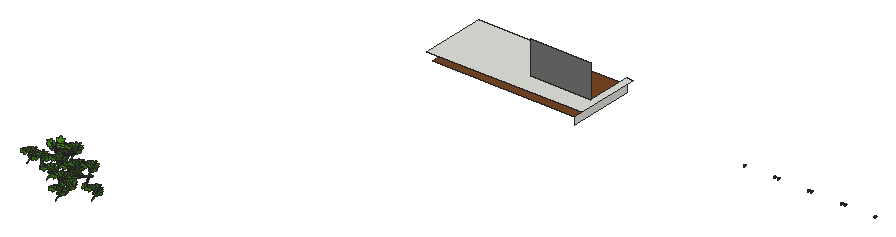
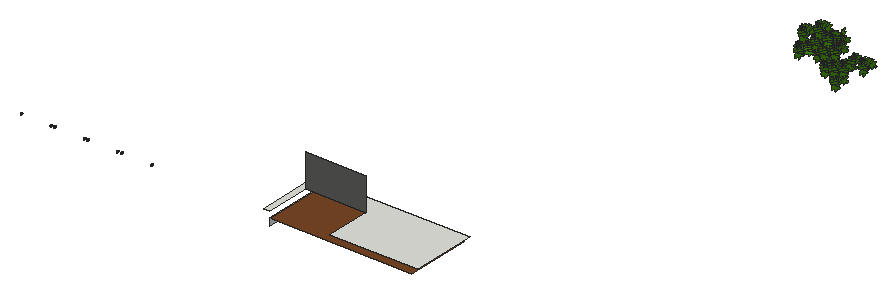
# SketchUp Ruby script. Lengths in inches.
U = 1.inch
M = Sketchup.active_model
def pt(a) = Geom::Point3d.new(a.map { |v| v * U })
def face(e, loops, mat)
  f = e.add_face(loops[0].map { |a| pt(a) })
  loops[1..].each { |l| e.add_face(l.map { |a| pt(a) }).erase! }
  f.material = f.back_material = mat if mat
  f
end
# faces: each face lists its corners as indices into pts; further lists are holes
def faces(e, pts, list, mat = nil) = list.each { |f| face(e, (f[0].is_a?(Array) ? f : [f]).map { |l| l.map { |i| pts[i] } }, mat) }
# xy, xz, yz: faces in a plane at the given z, y or x. An outline is a flat list of corners, or four numbers for a rectangle; further outlines are holes
def ring(l) = l.size == 4 ? [[l[0], l[1]], [l[2], l[1]], [l[2], l[3]], [l[0], l[3]]] : l.each_slice(2).to_a
def flat(e, list, mat, &to3) = list.each { |f| face(e, (f[0].is_a?(Array) ? f : [f]).map { |l| ring(l).map { |u, v| to3.(u, v) } }, mat) }
def xy(e, z, list, mat = nil) = flat(e, list, mat) { |x, y| [x, y, z] }
def xz(e, y, list, mat = nil) = flat(e, list, mat) { |x, z| [x, y, z] }
def yz(e, x, list, mat = nil) = flat(e, list, mat) { |y, z| [x, y, z] }
def lines(e, pts, list) = list.each { |a, b| e.add_line(pt(pts[a]), pt(pts[b])) }
# prism: a flat outline (further loops are holes) pulled along v
def prism(e, loops, v, mat = nil)
  f = face(e, loops, mat); d = Geom::Vector3d.new(v.map { |x| x * U })
  f.pushpull(f.normal.samedirection?(d) ? d.length : -d.length)
end
def box(e, o, s, mat = nil) = prism(e, [[o, [o[0] + s[0], o[1], o[2]], [o[0] + s[0], o[1] + s[1], o[2]], [o[0], o[1] + s[1], o[2]]]], [0, 0, s[2]], mat)
def at(x, y, z, deg = 0) = Geom::Transformation.translation(pt([x, y, z])) * Geom::Transformation.rotation(ORIGIN, Z_AXIS, deg.degrees)
def axes(o, x, y, z) = Geom::Transformation.new([*x, 0, *y, 0, *z, 0, *pt(o).to_a, 1])
def part(name) = M.definitions.add(name)
# library, detail: a bought-in or finely detailed component or shape, given as its bounding box
def library(name, o, s) = part(name).tap { |d| box(d.entities, o, s) }
def detail(e, o, s) = box(e.add_group.entities, o, s)
def put(e, d, t, mat = nil) = e.add_instance(d, t).tap { |i| i.material = mat if mat }
def group(e, t, mat = nil) = e.add_group.tap { |g| g.transformation = t; g.material = mat if mat }.entities
root = M.entities
M.materials.add("[Metal Seamed]").color = [116, 117, 113]
M.materials.add("[Wood Veneer 01]").color = [120, 70, 37]
M.materials.add("hojas").color = [70, 150, 19]
c1 = part("rama-acacia")
p = [[-13.53,0.69,-1.07],[-13.38,0.86,-0.98],[-13.61,0.85,-1.06],[-14.07,0.85,-1.21],[-15.17,0.86,-1.58],[-15.95,0.92,-1.83],
  [-16.01,1,-1.83],[-16.01,1.17,-1.78],[-16.07,1.93,-1.6],[-16.4,2.73,-1.5],[-16.65,3.06,-1.5],[-17.13,4.01,-1.41],
  [-17.78,4.7,-1.44],[-18.28,5.07,-1.51],[-18.57,5.18,-1.58],[-18.91,5.47,-1.62],[-19.07,5.48,-1.67],[-19.35,5.61,-1.73],
  [-19.51,5.64,-1.78],[-19.38,5.57,-1.75],[-19.33,5.5,-1.75],[-19.31,5.23,-1.82],[-19.38,5.08,-1.89],[-19.41,4.84,-1.96],
  [-19.36,4.59,-2.01],[-19.43,4.55,-2.04],[-19.36,4.15,-2.125],[-19.21,3.7,-2.19],[-18.875,3.1,-2.24],[-18.61,2.78,-2.24],
  [-17.83,2.19,-2.13],[-17.4375,1.85,-2.09],[-17.04,1.49,-2.05],[-16.61,1.24,-1.97],[-16.17,1.0625,-1.87],[-16.06,0.95,-1.86],
  [-16.06,0.91,-1.87],[-16.32,0.9,-1.96],[-16.7,0.88,-2.1],[-17.05,0.91,-2.21],[-17.61,1.15,-2.33],[-18.06,1.29,-2.45],
  [-18.88,1.53,-2.67],[-20.25,1.46,-3.15],[-20.59,1.49,-3.26],[-20.79,1.37,-3.36],[-21.08,1.2,-3.5],[-21.28,1.22,-3.5625],
  [-21.48,0.94,-3.71],[-21.79,0.5,-3.93],[-22.02,0.17,-4.1],[-22.11,0.05,-4.16],[-22.21,-0.02,-4.21],[-22.375,-0.05,-4.28],
  [-22.375,-0.07,-4.28],[-22.18,-0.09,-4.22],[-22.11,-0.07,-4.19],[-21.78,-0.1,-4.09],[-21.6,-0.18,-4.05],[-21.52,-0.27,-4.04],
  [-21.33,-0.33,-4],[-20.94,-0.54,-3.92],[-20.6875,-0.63,-3.86],[-20.54,-0.68,-3.82],[-20.42,-0.67,-3.78],[-20.09,-0.46,-3.61],
  [-19.8,-0.24,-3.45],[-19.21,-0.02,-3.19],[-18.48,0.08,-2.92],[-17.72,0.38,-2.58],[-17.4,0.5,-2.4375],[-16.93,0.75,-2.21],
  [-16.78,0.8,-2.15],[-16.1,0.83,-1.91],[-16.0625,0.81,-1.9],[-16.08,0.77,-1.91],[-16.27,0.72,-1.99],[-16.88,0.39,-2.29],
  [-17.1875,0.15,-2.46],[-17.27,0.02,-2.52],[-17.94,-0.52,-2.89],[-17.94,-0.59,-2.91],[-18.08,-0.68,-2.99],[-18.13,-0.86,-3.05],
  [-18.56,-1.55,-3.38],[-18.71,-2.11,-3.58],[-18.79,-2.61,-3.74],[-18.86,-2.84,-3.83],[-18.87,-3.07,-3.89],[-18.84,-3.22,-3.92],
  [-18.8,-3.26,-3.92],[-18.76,-3.47,-3.96],[-18.76,-3.6,-4],[-18.67,-3.8,-4.02],[-18.61,-3.92,-4.04],[-18.58,-4.11,-4.07],
  [-18.53,-4.18,-4.08],[-18.58,-4.35,-4.14],[-18.65,-4.43,-4.18],[-18.72,-4.51,-4.23],[-18.8125,-4.51,-4.26],[-18.8125,-4.53,-4.26],
  [-18.72,-4.54,-4.24],[-18.66,-4.49,-4.21],[-18.58,-4.43,-4.16],[-18.35,-4.23,-4.03],[-18.32,-4.17,-4],[-18.22,-4.125,-3.95],
  [-18.1,-4,-3.88],[-17.79,-3.72,-3.7],[-17.68,-3.51,-3.61],[-17.32,-3.13,-3.38],[-17.24,-2.94,-3.31],[-16.78,-2.12,-2.93],
  [-16.48,-1.78,-2.73],[-16.3,-1.28,-2.54],[-16.05,-0.75,-2.3125],[-15.89,-0.2,-2.11],[-15.89,0.39,-1.95],[-15.96,0.79,-1.87],
  [-15.91,0.82,-1.84],[-15.27,0.8,-1.63],[-14.18,0.76,-1.27],[-13.78,0.73,-1.15],[-13.78,0.67,-1.16],[-14.23,0.54,-1.35],
  [-14.65,0.33,-1.55],[-14.97,0.02,-1.74],[-15.25,-0.36,-1.9375],[-15.57,-0.72,-2.14],[-15.96,-1.64,-2.52],[-16.2,-2.51,-2.84],
  [-16.2,-3.12,-3],[-16.14,-3.41,-3.06],[-16.1,-3.75,-3.14],[-16.1,-4.09,-3.23],[-16.2,-4.25,-3.3],[-16.2,-4.28,-3.3125],
  [-16.08,-4.19,-3.24],[-15.98,-4.08,-3.18],[-15.96,-3.94,-3.14],[-15.96,-3.8125,-3.1],[-15.9,-3.72,-3.06],[-15.68,-3.55,-2.9375],
  [-15.51,-3.49,-2.86],[-15.3,-3.33,-2.75],[-15.23,-3.17,-2.68],[-15.01,-3.03,-2.57],[-14.875,-2.83,-2.47],[-14.6,-2.59,-2.3125],
  [-14.4,-2.27,-2.16],[-14.12,-1.6,-1.89],[-13.91,-1.1,-1.68],[-13.67,-0.83,-1.53],[-13.53,-0.45,-1.38],[-13.53,0.67,-1.08],
  [-12.41,6.01,0.65],[-12.44,6.14,0.68],[-12.41,6.29,0.73],[-12.43,6.29,0.73],[-12.44,6.26,0.72],[-12.47,6.15,0.68],
  [-12.49,6.07,0.66],[-12.57,5.75,0.55],[-12.67,5.36,0.43],[-12.79,4.875,0.28],[-12.83,4.52,0.18],[-12.83,3.99,0.04],
  [-12.73,3.11,-0.18],[-12.58,2.52,-0.3125],[-12.3,1.97,-0.41],[-11.88,1.51,-0.46],[-11.37,1.0625,-0.48],[-10.75,0.75,-0.45],
  [-10.75,0.68,-0.47],[-12.55,0.7,-0.79],[-13.21,0.79,-0.89],[-13.2,0.67,-0.92],[-12.56,0.62,-0.82],[-11.15,0.56,-0.58],
  [-10.79,0.54,-0.52],[-10.72,0.52,-0.51],[-10.72,0.5,-0.52],[-10.87,0.47,-0.55],[-11.14,0.41,-0.62],[-11.39,0.27,-0.7],
  [-11.625,-0.01,-0.82],[-11.8,-0.43,-0.96],[-11.83,-0.57,-1],[-12.02,-1.08,-1.17],[-12.1,-1.39,-1.27],[-12.17,-1.95,-1.4375],
  [-12.17,-2.77,-1.65],[-12.09,-3.59,-1.86],[-11.86,-4.26,-2],[-11.8125,-4.4,-2.03],[-11.84,-4.49,-2.05],[-11.91,-4.6,-2.1],
  [-11.97,-4.65,-2.12],[-11.98,-4.67,-2.13],[-11.92,-4.65,-2.11],[-11.84,-4.59,-2.08],[-11.77,-4.52,-2.05],[-11.74,-4.47,-2.03],
  [-11.37,-4.3125,-1.92],[-10.95,-4.0625,-1.78],[-10.82,-3.89,-1.71],[-10.64,-3.57,-1.59],[-10.41,-3.05,-1.41],[-10.27,-2.73,-1.3],
  [-10.07,-1.88,-1.03],[-10.15,-0.71,-0.73],[-10.31,-0.1,-0.6],[-10.5,0.4,-0.5],[-10.5,0.48,-0.48],[-10.44,0.53,-0.45],
  [-10.39,0.64,-0.42],[-10.52,0.73,-0.42],[-10.44,0.93,-0.35],[-10.44,1.2,-0.28],[-10.32,1.47,-0.18],[-10.48,2.6875,0.12],
  [-10.43,2.96,0.2],[-10.75,3.87,0.38],[-11.26,4.93,0.57],[-11.8,5.54,0.64],[-12.37,5.93,0.64],[-7.78,0.19,-0.06],
  [-7.78,0.25,-0.04],[-7.75,0.39,0],[-7.89,0.4,-0.02],[-7.96,0.46,-0.02],[-7.96,0.49,-0.01],[-7.76,0.62,0.06],
  [-7.53,0.99,0.2],[-7.31,1.78,0.45],[-7.31,2.74,0.71],[-7.63,3.6875,0.9],[-8.02,4.57,1.07],[-8.66,5.23,1.13],
  [-8.83,5.4,1.14],[-8.92,5.54,1.16],[-9.1,5.64,1.16],[-9.08,5.6,1.15],[-9.02,5.56,1.15],[-8.94,5.46,1.14],
  [-8.9,5.37,1.12],[-8.9375,5.25,1.08],[-9.14,4.92,0.96],[-9.31,4.5625,0.83],[-9.39,3.73,0.6],[-9.44,2.76,0.32],
  [-9.23,1.59,0.05],[-8.82,0.9,-0.06],[-8.36,0.59,-0.0625],[-8.14,0.51,-0.04],[-8.05,0.48,-0.03],[-8.05,0.46,-0.04],
  [-8.12,0.43,-0.06],[-10.1,0.49,-0.4],[-8.22,0.3125,-0.11],[-8.22,0.25,-0.125],[-8.53,0.13,-0.21],[-8.8,-0.16,-0.34],
  [-8.96,-0.61,-0.49],[-8.96,-0.87,-0.56],[-9.16,-1.42,-0.74],[-9.13,-1.77,-0.83],[-9.09,-1.83,-0.84],[-9.125,-1.92,-0.87],
  [-9.125,-2.13,-0.93],[-9.08,-2.23,-0.95],[-9.15,-2.39,-1],[-9.11,-2.67,-1.07],[-9.03,-2.86,-1.11],[-9.07,-3.03,-1.16],
  [-8.97,-3.23,-1.19],[-8.93,-3.44,-1.24],[-8.93,-3.71,-1.32],[-8.79,-4.05,-1.38],[-8.7,-4.25,-1.42],[-8.7,-4.39,-1.46],
  [-8.76,-4.53,-1.5],[-8.77,-4.65,-1.54],[-8.64,-4.55,-1.49],[-8.27,-4.22,-1.33],[-8.1875,-4.06,-1.27],[-8.07,-3.98,-1.23],
  [-7.98,-3.79,-1.17],[-7.79,-3.59,-1.08],[-7.64,-3.3,-0.97],[-7.64,-3.25,-0.96],[-7.59,-3.21,-0.9375],[-7.52,-2.93,-0.85],
  [-7.52,-2.85,-0.83],[-7.47,-2.81,-0.81],[-7.3,-2.09,-0.59],[-7.32,-2.01,-0.57],[-7.27,-1.95,-0.54],[-7.1875,-1.57,-0.42],
  [-7.17,-1.46,-0.39],[-7.17,-1.16,-0.3125],[-7.23,-0.61,-0.17],[-7.49,-0.15,-0.1],[-13.39,-0.07,-1.23],[-13.39,0.25,-1.14],
  [-13.49,0.5625,-1.09],[-13.8,1.01,-1.08],[-13.61,0.91,-1.04],[-13.38,0.92,-0.96],[-13.32,1.03,-0.91],[-13.32,1.35,-0.82],
  [-13.28,1.49,-0.77],[-13.28,1.99,-0.64],[-13.44,2.67,-0.51],[-13.72,3.31,-0.43],[-13.93,3.71,-0.4],[-14.1,4.39,-0.27],
  [-14.5625,5.06,-0.25],[-14.89,5.62,-0.21],[-15.33,6.1,-0.23],[-15.65,6.8,-0.15],[-15.79,6.89,-0.18],[-15.61,6.52,-0.22],
  [-15.51,6.32,-0.24],[-15.45,6.28,-0.23],[-15.52,6,-0.32],[-15.63,5.6875,-0.45],[-15.77,4.97,-0.68],[-15.7,4.25,-0.85],
  [-15.46,3,-1.11],[-15,2.03,-1.21],[-14.3,1.29,-1.17],[-4.5625,0.33,0.09],[-4.22,0.49,0.13],[-4,0.7,0.1875],
  [-3.86,0.99,0.26],[-3.77,1.41,0.38],[-3.7,1.73,0.46],[-3.77,1.99,0.53],[-3.85,2.17,0.58],[-3.88,2.57,0.6875],
  [-3.98,2.9,0.78],[-4.0625,2.97,0.8],[-4.1,3.14,0.84],[-4.1875,3.25,0.87],[-4.27,3.55,0.95],[-4.31,3.71,0.99],
  [-4.42,3.9,1.04],[-4.625,4.2,1.125],[-4.72,4.39,1.18],[-4.89,4.57,1.23],[-4.98,4.73,1.27],[-5,4.72,1.26],
  [-5.01,4.51,1.21],[-4.96,4.32,1.16],[-4.97,4.27,1.14],[-5.14,3.78,1.01],[-5.3,3.39,0.91],[-5.44,2.76,0.74],
  [-5.5,2.09,0.56],[-5.57,1.78,0.48],[-5.57,1.42,0.38],[-5.57,1.09,0.29],[-5.47,0.72,0.19],[-5.22,0.44,0.12],
  [-4.93,0.27,0.07],[-4.76,0.22,0.06],[-4.76,0.18,0.05],[-4.83,0.16,0.04],[-5.26,0,0],[-5.34,-0.04,-0.01],
  [-5.47,-0.22,-0.06],[-5.51,-0.6,-0.16],[-5.42,-1.09,-0.29],[-5.28,-1.49,-0.4],[-5.21,-1.87,-0.5],[-5.11,-2.15,-0.57],
  [-5.08,-2.34,-0.63],[-5.01,-2.47,-0.66],[-4.96,-2.69,-0.72],[-4.86,-2.9375,-0.79],[-4.84,-3.07,-0.82],[-4.77,-3.18,-0.85],
  [-4.74,-3.43,-0.92],[-4.7,-3.71,-0.99],[-4.62,-3.89,-1.04],[-4.58,-3.98,-1.07],[-4.58,-3.83,-1.03],[-4.51,-3.67,-0.98],
  [-4.3,-3.32,-0.89],[-4.16,-3.09,-0.83],[-4.16,-2.98,-0.8],[-4.11,-2.92,-0.78],[-4.02,-2.8,-0.75],[-3.95,-2.59,-0.69],
  [-3.95,-2.33,-0.625],[-3.86,-2.26,-0.6],[-3.86,-2.02,-0.54],[-3.86,-1.44,-0.39],[-3.94,-1.22,-0.33],[-3.94,-1.08,-0.29],
  [-4,-0.96,-0.26],[-4,-0.87,-0.23],[-4.0625,-0.8125,-0.22],[-4.16,-0.54,-0.14],[-4.39,-0.24,-0.06],[-4.61,-0.08,-0.02],
  [-4.77,-0.03,-0.01],[-4.77,-0.01,0],[-4.65,-0.01,0],[-4.61,0.19,0.05],[-4.66,0.23,0.0625],[-4.63,0.29,0.08],
  [-4.07,0.17,0.04],[0,-0.24,-0.06],[0,0,0],[-0.5,0.04,0.01],[-1.58,0.08,0.02],[-13.78,0.67,-1.08]]
faces(c1.entities,p,[[0,1,2,3,4,5,6,7,8,9,10,11,12,13,14,15,16,17,18,19,20,21,22,23,24,25,26,27,28,29,30,31,32,33,34,35,36,37,38,39,40,41,42,43,44,45,46,47,48,49,50,51,52,53,54,55,56,57,58,59,60,61,62,63,64,65,66,67,68,69,70,71,72,73,74,75,76,77,78,79,80,81,82,83,84,85,86,87,88,89,90,91,92,93,94,95,96,97,98,99,100,101,102,103,104,105,106,107,108,109,110,111,112,113,114,115,116,117,118,119,120,121,122,123,124,125,126,127,128,129,130,131,132,133,134,135,136,137,138,139,140,141,142,143,144,145,146,147,148,149,150,151,152,153,154,155],[156,157,158,159,160,161,162,163,164,165,166,167,168,169,170,171,172,173,174,175,176,177,178,179,180,181,182,183,184,185,186,187,188,189,190,191,192,193,194,195,196,197,198,199,200,201,202,203,204,205,206,207,208,209,210,211,212,213,214,215,216,217,218,219,220,221,222,223,224,225,226],[227,228,229,230,231,232,233,234,235,236,237,238,239,240,241,242,243,244,245,246,247,248,249,250,251,252,253,254,255,256,257,258,216,215,259,260,261,262,263,264,265,266,267,268,269,270,271,272,273,274,275,276,277,278,279,280,281,282,283,284,285,286,287,288,289,290,291,292,293,294,295,296,297,298,299,300,301,302,303],[154,304,305,306,155],[307,308,1,309,310,311,312,313,314,315,316,317,318,319,320,321,322,323,324,325,326,327,328,329,330,331,332],[333,334,335,336,337,338,339,340,341,342,343,344,345,346,347,348,349,350,351,352,353,354,355,356,357,358,359,360,361,362,363,364,365,366,367,368,369,370,371,372,373,374,375,376,377,378,379,380,381,382,383,384,385,386,387,388,389,390,391,392,393,394,395,396,397,398,399,400,401,402,403,404,405,406,407,408,409,410,411,412,413],[0,177,1],[308,2,1],
  [176,1,177],[414,411,410,415,416,417,418],[228,370,229],[369,229,370]],"hojas")
lines(c1.entities,p,[[155,419]])
c2 = part("Group\#150")
put(c2.entities,c1,axes([10.13,10.27,0],[0.45315,0.21131,0],[-0.21131,0.45315,0],[0,0,0.5]))
put(c2.entities,c1,axes([10.13,10.27,0],[0.11638,0.47539,0.10227],[-0.48087,0.12813,-0.0484],[-0.07223,-0.08709,0.48703]))
put(c2.entities,c1,axes([9.58,10.26,-0.7],[0.1449,0.38901,-0.2787],[-0.10883,0.31035,0.37662],[0.46601,-0.04848,0.17461]))
c3 = part("Group\#151")
put(c3.entities,c2,axes([24.99,4.24,9.59],[0.78856,0.61496,0],[0.01473,-0.01889,0.99971],[0.61478,-0.78833,-0.02396]))
put(c3.entities,c2,axes([39.5,6.625,12.55],[0.6544,0.49291,0.57341],[-0.44023,-0.3682,0.81892],[0.61478,-0.78833,-0.02396]))
put(c3.entities,c2,axes([32.34,3.7,6.88],[0.78856,0.61496,0],[0.01473,-0.01889,0.99971],[0.61478,-0.78833,-0.02396]))
put(c3.entities,c2,axes([43.14,6.65,17.54],[0.78856,0.61496,0],[0.35273,-0.4523,0.81915],[0.50374,-0.64595,-0.57358]))
put(c3.entities,c2,axes([12.2,6.2,16.68],[0.7209,0.54936,0.4225],[-0.31991,-0.27701,0.90605],[0.61478,-0.78833,-0.02396]))
put(c3.entities,c2,axes([49.9375,3.79,26.09],[0.78856,0.61496,0],[0.01473,-0.01889,0.99971],[0.61478,-0.78833,-0.02396]))
put(c3.entities,c2,axes([36.11,4.9375,33.94],[0.78856,0.61496,0],[0.01473,-0.01889,0.99971],[0.61478,-0.78833,-0.02396]))
put(c3.entities,c2,axes([39.61,3.79,23.47],[0.78856,0.61496,0],[0.01473,-0.01889,0.99971],[0.61478,-0.78833,-0.02396]))
put(c3.entities,c2,axes([25.59,6.5625,46.47],[-0.40704,-0.29112,-0.86578],[0.67555,0.54201,-0.49986],[0.61478,-0.78833,-0.02396]))
put(c3.entities,c2,axes([54.97,1.98,11.65],[0.78856,0.61496,0],[0.01473,-0.01889,0.99971],[0.61478,-0.78833,-0.02396]))
put(c3.entities,c2,axes([32.97,3.79,19.14],[0.78856,0.61496,0],[0.01473,-0.01889,0.99971],[0.61478,-0.78833,-0.02396]))
put(c3.entities,c2,axes([24.24,3.79,21.99],[0.78856,0.61496,0],[0.01473,-0.01889,0.99971],[0.61478,-0.78833,-0.02396]))
put(c3.entities,c2,axes([16.86,4.24,12.3],[0.78856,0.61496,0],[0.01473,-0.01889,0.99971],[0.61478,-0.78833,-0.02396]))
put(c3.entities,c2,axes([1.23,3.9375,19.07],[0.78856,0.61496,0],[0.01473,-0.01889,0.99971],[0.61478,-0.78833,-0.02396]))
put(c3.entities,c2,axes([29.05,5.25,29.11],[0.78856,0.61496,0],[0.21033,-0.2697,0.93969],[0.57787,-0.741,-0.34202]))
put(c3.entities,c2,axes([24.16,3.79,-0.1],[0.78856,0.61496,0],[0.01473,-0.01889,0.99971],[0.61478,-0.78833,-0.02396]))
xy(root,114.25,[[3002.95,732.28,3250.36,845.35]],"[Wood Veneer 01]")
xy(root,125.1875,[[2992.01,732.28,3261.3,732.28,3261.3,845.35,3249.37,845.35,3249.37,767.72,3145.18,767.72,3145.18,845.35,2992.01,845.35]])
xz(root,767.72,[[3145.18,125.1875,3249.37,183.3125]],"[Metal Seamed]")
xz(root,799.91,[[3491.38,91.63,3491.67,91.67,3491.94,91.78,3492.17,91.96,3492.35,92.19,3492.46,92.46,3492.5,92.75,3492.46,93.04,3492.35,93.32,3492.17,93.55,3491.94,93.73,3491.67,93.84,3491.38,93.88,3491.09,93.84,3490.82,93.73,3490.58,93.55,3490.4,93.32,3490.29,93.04,3490.25,92.75,3490.29,92.46,3490.4,92.19,3490.58,91.96,3490.82,91.78,3491.09,91.67],[3543.57,91.63,3543.86,91.67,3544.13,91.78,3544.36,91.96,3544.54,92.19,3544.65,92.46,3544.69,92.75,3544.65,93.04,3544.54,93.32,3544.36,93.55,3544.13,93.73,3543.86,93.84,3543.57,93.88,3543.27,93.84,3543,93.73,3542.77,93.55,3542.59,93.32,3542.48,93.04,3542.44,92.75,3542.48,92.46,3542.59,92.19,3542.77,91.96,3543,91.78,3543.27,91.67],[3550.37,91.63,3550.66,91.67,3550.93,91.78,3551.16,91.96,3551.34,92.19,3551.45,92.46,3551.49,92.75,3551.45,93.04,3551.34,93.32,3551.16,93.55,3550.93,93.73,3550.66,93.84,3550.37,93.88,3550.08,93.84,3549.8,93.73,3549.57,93.55,3549.39,93.32,3549.28,93.04,3549.24,92.75,3549.28,92.46,3549.39,92.19,3549.57,91.96,3549.8,91.78,3550.08,91.67],[3602.55,91.63,3602.85,91.67,3603.12,91.78,3603.35,91.96,3603.53,92.19,3603.64,92.46,3603.68,92.75,3603.64,93.04,3603.53,93.32,3603.35,93.55,3603.12,93.73,3602.85,93.84,3602.55,93.88,3602.26,93.84,3601.99,93.73,3601.76,93.55,3601.58,93.32,3601.47,93.04,3601.43,92.75,3601.47,92.46,3601.58,92.19,3601.76,91.96,3601.99,91.78,3602.26,91.67],[3608.54,91.63,3608.83,91.67,3609.1,91.78,3609.34,91.96,3609.52,92.19,3609.63,92.46,3609.67,92.75,3609.63,93.04,3609.52,93.32,3609.34,93.55,3609.1,93.73,3608.83,93.84,3608.54,93.88,3608.25,93.84,3607.98,93.73,3607.75,93.55,3607.57,93.32,3607.46,93.04,3607.42,92.75,3607.46,92.46,3607.57,92.19,3607.75,91.96,3607.98,91.78,3608.25,91.67],
  [3660.73,91.63,3661.02,91.67,3661.29,91.78,3661.53,91.96,3661.7,92.19,3661.82,92.46,3661.85,92.75,3661.82,93.04,3661.7,93.32,3661.53,93.55,3661.29,93.73,3661.02,93.84,3660.73,93.88,3660.4375,93.84,3660.17,93.73,3659.93,93.55,3659.76,93.32,3659.64,93.04,3659.6,92.75,3659.64,92.46,3659.76,92.19,3659.93,91.96,3660.17,91.78,3660.4375,91.67],[3666.84,91.63,3667.13,91.67,3667.41,91.78,3667.64,91.96,3667.82,92.19,3667.93,92.46,3667.97,92.75,3667.93,93.04,3667.82,93.32,3667.64,93.55,3667.41,93.73,3667.13,93.84,3666.84,93.88,3666.55,93.84,3666.28,93.73,3666.05,93.55,3665.87,93.32,3665.76,93.04,3665.72,92.75,3665.76,92.46,3665.87,92.19,3666.05,91.96,3666.28,91.78,3666.55,91.67],[3719.03,91.63,3719.32,91.67,3719.59,91.78,3719.83,91.96,3720,92.19,3720.12,92.46,3720.16,92.75,3720.12,93.04,3720,93.32,3719.83,93.55,3719.59,93.73,3719.32,93.84,3719.03,93.88,3718.74,93.84,3718.47,93.73,3718.24,93.55,3718.06,93.32,3717.94,93.04,3717.91,92.75,3717.94,92.46,3718.06,92.19,3718.24,91.96,3718.47,91.78,3718.74,91.67]])
yz(root,3250.36,[[732.28,101.375,845.35,114.25]])
p = [[3491.09,801.78,91.67],[3491.38,801.78,91.63],[3491.38,799.91,91.63],[3491.09,799.91,91.67],[3491.67,801.78,91.67],[3491.67,799.91,91.67],
  [3543.27,801.78,91.67],[3543.57,801.78,91.63],[3543.57,799.91,91.63],[3543.27,799.91,91.67],[3543.86,801.78,91.67],[3543.86,799.91,91.67],
  [3550.08,801.78,91.67],[3550.37,801.78,91.63],[3550.37,799.91,91.63],[3550.08,799.91,91.67],[3550.66,801.78,91.67],[3550.66,799.91,91.67],
  [3602.26,801.78,91.67],[3602.55,801.78,91.63],[3602.55,799.91,91.63],[3602.26,799.91,91.67],[3602.85,801.78,91.67],[3602.85,799.91,91.67],
  [3608.25,801.78,91.67],[3608.54,801.78,91.63],[3608.54,799.91,91.63],[3608.25,799.91,91.67],[3608.83,801.78,91.67],[3608.83,799.91,91.67],
  [3660.4375,801.78,91.67],[3660.73,801.78,91.63],[3660.73,799.91,91.63],[3660.4375,799.91,91.67],[3661.02,801.78,91.67],[3661.02,799.91,91.67],
  [3666.55,801.78,91.67],[3666.84,801.78,91.63],[3666.84,799.91,91.63],[3666.55,799.91,91.67],[3667.13,801.78,91.67],[3667.13,799.91,91.67],
  [3718.74,801.78,91.67],[3719.03,801.78,91.63],[3719.03,799.91,91.63],[3718.74,799.91,91.67],[3719.32,801.78,91.67],[3719.32,799.91,91.67],
  [3490.82,801.78,91.78],[3490.82,799.91,91.78],[3491.94,801.78,91.78],[3491.94,799.91,91.78],[3543,801.78,91.78],[3543,799.91,91.78],
  [3544.13,801.78,91.78],[3544.13,799.91,91.78],[3549.8,801.78,91.78],[3549.8,799.91,91.78],[3550.93,801.78,91.78],[3550.93,799.91,91.78],
  [3601.99,801.78,91.78],[3601.99,799.91,91.78],[3603.12,801.78,91.78],[3603.12,799.91,91.78],[3607.98,801.78,91.78],[3607.98,799.91,91.78],
  [3609.1,801.78,91.78],[3609.1,799.91,91.78],[3660.17,801.78,91.78],[3660.17,799.91,91.78],[3661.29,801.78,91.78],[3661.29,799.91,91.78],
  [3666.28,801.78,91.78],[3666.28,799.91,91.78],[3667.41,801.78,91.78],[3667.41,799.91,91.78],[3718.47,801.78,91.78],[3718.47,799.91,91.78],
  [3719.59,801.78,91.78],[3719.59,799.91,91.78],[3490.58,801.78,91.96],[3490.58,799.91,91.96],[3492.17,801.78,91.96],[3492.17,799.91,91.96],
  [3542.77,801.78,91.96],[3542.77,799.91,91.96],[3544.36,801.78,91.96],[3544.36,799.91,91.96],[3549.57,801.78,91.96],[3549.57,799.91,91.96],
  [3551.16,801.78,91.96],[3551.16,799.91,91.96],[3601.76,801.78,91.96],[3601.76,799.91,91.96],[3603.35,801.78,91.96],[3603.35,799.91,91.96],
  [3607.75,801.78,91.96],[3607.75,799.91,91.96],[3609.34,801.78,91.96],[3609.34,799.91,91.96],[3659.93,801.78,91.96],[3659.93,799.91,91.96],
  [3661.53,801.78,91.96],[3661.53,799.91,91.96],[3666.05,801.78,91.96],[3666.05,799.91,91.96],[3667.64,801.78,91.96],[3667.64,799.91,91.96],
  [3718.24,801.78,91.96],[3718.24,799.91,91.96],[3719.83,801.78,91.96],[3719.83,799.91,91.96],[3490.4,801.78,92.19],[3490.4,799.91,92.19],
  [3492.35,801.78,92.19],[3492.35,799.91,92.19],[3542.59,801.78,92.19],[3542.59,799.91,92.19],[3544.54,801.78,92.19],[3544.54,799.91,92.19],
  [3549.39,801.78,92.19],[3549.39,799.91,92.19],[3551.34,801.78,92.19],[3551.34,799.91,92.19],[3601.58,801.78,92.19],[3601.58,799.91,92.19],
  [3603.53,801.78,92.19],[3603.53,799.91,92.19],[3607.57,801.78,92.19],[3607.57,799.91,92.19],[3609.52,801.78,92.19],[3609.52,799.91,92.19],
  [3659.76,801.78,92.19],[3659.76,799.91,92.19],[3661.7,801.78,92.19],[3661.7,799.91,92.19],[3665.87,801.78,92.19],[3665.87,799.91,92.19],
  [3667.82,801.78,92.19],[3667.82,799.91,92.19],[3718.06,801.78,92.19],[3718.06,799.91,92.19],[3720,801.78,92.19],[3720,799.91,92.19],
  [3490.29,801.78,92.46],[3490.29,799.91,92.46],[3492.46,801.78,92.46],[3492.46,799.91,92.46],[3542.48,801.78,92.46],[3542.48,799.91,92.46],
  [3544.65,801.78,92.46],[3544.65,799.91,92.46],[3549.28,801.78,92.46],[3549.28,799.91,92.46],[3551.45,801.78,92.46],[3551.45,799.91,92.46],
  [3601.47,801.78,92.46],[3601.47,799.91,92.46],[3603.64,801.78,92.46],[3603.64,799.91,92.46],[3607.46,801.78,92.46],[3607.46,799.91,92.46],
  [3609.63,801.78,92.46],[3609.63,799.91,92.46],[3659.64,801.78,92.46],[3659.64,799.91,92.46],[3661.82,801.78,92.46],[3661.82,799.91,92.46],
  [3665.76,801.78,92.46],[3665.76,799.91,92.46],[3667.93,801.78,92.46],[3667.93,799.91,92.46],[3717.94,801.78,92.46],[3717.94,799.91,92.46],
  [3720.12,801.78,92.46],[3720.12,799.91,92.46],[3490.25,801.78,92.75],[3490.25,799.91,92.75],[3492.5,801.78,92.75],[3492.5,799.91,92.75],
  [3542.44,801.78,92.75],[3542.44,799.91,92.75],[3544.69,801.78,92.75],[3544.69,799.91,92.75],[3549.24,801.78,92.75],[3549.24,799.91,92.75],
  [3551.49,801.78,92.75],[3551.49,799.91,92.75],[3601.43,801.78,92.75],[3601.43,799.91,92.75],[3603.68,801.78,92.75],[3603.68,799.91,92.75],
  [3607.42,801.78,92.75],[3607.42,799.91,92.75],[3609.67,801.78,92.75],[3609.67,799.91,92.75],[3659.6,801.78,92.75],[3659.6,799.91,92.75],
  [3665.72,801.78,92.75],[3665.72,799.91,92.75],[3667.97,801.78,92.75],[3667.97,799.91,92.75],[3717.91,801.78,92.75],[3717.91,799.91,92.75],
  [3720.16,801.78,92.75],[3720.16,799.91,92.75],[3490.29,801.78,93.04],[3490.29,799.91,93.04],[3492.46,801.78,93.04],[3492.46,799.91,93.04],
  [3542.48,801.78,93.04],[3542.48,799.91,93.04],[3544.65,801.78,93.04],[3544.65,799.91,93.04],[3549.28,801.78,93.04],[3549.28,799.91,93.04],
  [3551.45,801.78,93.04],[3551.45,799.91,93.04],[3601.47,801.78,93.04],[3601.47,799.91,93.04],[3603.64,801.78,93.04],[3603.64,799.91,93.04],
  [3607.46,801.78,93.04],[3607.46,799.91,93.04],[3609.63,801.78,93.04],[3609.63,799.91,93.04],[3659.64,801.78,93.04],[3659.64,799.91,93.04],
  [3665.76,801.78,93.04],[3665.76,799.91,93.04],[3667.93,801.78,93.04],[3667.93,799.91,93.04],[3717.94,801.78,93.04],[3717.94,799.91,93.04],
  [3720.12,801.78,93.04],[3720.12,799.91,93.04],[3490.4,801.78,93.32],[3490.4,799.91,93.32],[3492.35,801.78,93.32],[3492.35,799.91,93.32],
  [3542.59,801.78,93.32],[3542.59,799.91,93.32],[3544.54,801.78,93.32],[3544.54,799.91,93.32],[3549.39,801.78,93.32],[3549.39,799.91,93.32],
  [3551.34,801.78,93.32],[3551.34,799.91,93.32],[3601.58,801.78,93.32],[3601.58,799.91,93.32],[3603.53,801.78,93.32],[3603.53,799.91,93.32],
  [3607.57,801.78,93.32],[3607.57,799.91,93.32],[3609.52,801.78,93.32],[3609.52,799.91,93.32],[3659.76,801.78,93.32],[3659.76,799.91,93.32],
  [3665.87,801.78,93.32],[3665.87,799.91,93.32],[3667.82,801.78,93.32],[3667.82,799.91,93.32],[3718.06,801.78,93.32],[3718.06,799.91,93.32],
  [3720,801.78,93.32],[3720,799.91,93.32],[3490.58,801.78,93.55],[3490.58,799.91,93.55],[3492.17,801.78,93.55],[3492.17,799.91,93.55],
  [3542.77,801.78,93.55],[3542.77,799.91,93.55],[3544.36,801.78,93.55],[3544.36,799.91,93.55],[3549.57,801.78,93.55],[3549.57,799.91,93.55],
  [3551.16,801.78,93.55],[3551.16,799.91,93.55],[3601.76,801.78,93.55],[3601.76,799.91,93.55],[3603.35,801.78,93.55],[3603.35,799.91,93.55],
  [3607.75,801.78,93.55],[3607.75,799.91,93.55],[3609.34,801.78,93.55],[3609.34,799.91,93.55],[3659.93,801.78,93.55],[3659.93,799.91,93.55],
  [3661.7,801.78,93.32],[3661.53,801.78,93.55],[3661.53,799.91,93.55],[3661.7,799.91,93.32],[3666.05,801.78,93.55],[3666.05,799.91,93.55],
  [3667.64,801.78,93.55],[3667.64,799.91,93.55],[3718.24,801.78,93.55],[3718.24,799.91,93.55],[3719.83,801.78,93.55],[3719.83,799.91,93.55],
  [3490.82,801.78,93.73],[3490.82,799.91,93.73],[3491.94,801.78,93.73],[3491.94,799.91,93.73],[3543,801.78,93.73],[3543,799.91,93.73],
  [3544.13,801.78,93.73],[3544.13,799.91,93.73],[3549.8,801.78,93.73],[3549.8,799.91,93.73],[3550.93,801.78,93.73],[3550.93,799.91,93.73],
  [3601.99,801.78,93.73],[3601.99,799.91,93.73],[3603.12,801.78,93.73],[3603.12,799.91,93.73],[3607.98,801.78,93.73],[3607.98,799.91,93.73],
  [3609.1,801.78,93.73],[3609.1,799.91,93.73],[3660.17,801.78,93.73],[3660.17,799.91,93.73],[3661.29,801.78,93.73],[3661.29,799.91,93.73],
  [3666.28,801.78,93.73],[3666.28,799.91,93.73],[3667.41,801.78,93.73],[3667.41,799.91,93.73],[3718.47,801.78,93.73],[3718.47,799.91,93.73],
  [3719.59,801.78,93.73],[3719.59,799.91,93.73],[3491.09,801.78,93.84],[3491.09,799.91,93.84],[3491.67,801.78,93.84],[3491.67,799.91,93.84],
  [3543.27,801.78,93.84],[3543.27,799.91,93.84],[3543.86,801.78,93.84],[3543.86,799.91,93.84],[3550.08,801.78,93.84],[3550.08,799.91,93.84],
  [3550.66,801.78,93.84],[3550.66,799.91,93.84],[3602.26,801.78,93.84],[3602.26,799.91,93.84],[3602.85,801.78,93.84],[3602.85,799.91,93.84],
  [3608.25,801.78,93.84],[3608.25,799.91,93.84],[3608.83,801.78,93.84],[3608.83,799.91,93.84],[3660.4375,801.78,93.84],[3660.4375,799.91,93.84],
  [3661.02,801.78,93.84],[3661.02,799.91,93.84],[3666.55,801.78,93.84],[3666.55,799.91,93.84],[3667.13,801.78,93.84],[3667.13,799.91,93.84],
  [3718.74,801.78,93.84],[3718.74,799.91,93.84],[3719.32,801.78,93.84],[3719.32,799.91,93.84],[3491.38,801.78,93.88],[3491.38,799.91,93.88],
  [3543.57,801.78,93.88],[3543.57,799.91,93.88],[3550.37,801.78,93.88],[3550.37,799.91,93.88],[3602.55,801.78,93.88],[3602.55,799.91,93.88],
  [3608.54,801.78,93.88],[3608.54,799.91,93.88],[3660.73,801.78,93.88],[3660.73,799.91,93.88],[3666.84,801.78,93.88],[3666.84,799.91,93.88],
  [3719.03,801.78,93.88],[3719.03,799.91,93.88]]
faces(root,p,[[0,1,2,3],[1,4,5,2],[6,7,8,9],[7,10,11,8],[12,13,14,15],[13,16,17,14],[18,19,20,21],[19,22,23,20],
  [24,25,26,27],[25,28,29,26],[30,31,32,33],[31,34,35,32],[36,37,38,39],[37,40,41,38],[42,43,44,45],[43,46,47,44],
  [48,0,3,49],[4,50,51,5],[52,6,9,53],[10,54,55,11],[56,12,15,57],[16,58,59,17],[60,18,21,61],[22,62,63,23],
  [64,24,27,65],[28,66,67,29],[68,30,33,69],[34,70,71,35],[72,36,39,73],[40,74,75,41],[76,42,45,77],[46,78,79,47],
  [80,48,49,81],[50,82,83,51],[84,52,53,85],[54,86,87,55],[88,56,57,89],[58,90,91,59],[92,60,61,93],[62,94,95,63],
  [96,64,65,97],[66,98,99,67],[100,68,69,101],[70,102,103,71],[104,72,73,105],[74,106,107,75],[108,76,77,109],[78,110,111,79],
  [112,80,81,113],[82,114,115,83],[116,84,85,117],[86,118,119,87],[120,88,89,121],[90,122,123,91],[124,92,93,125],[94,126,127,95],
  [128,96,97,129],[98,130,131,99],[132,100,101,133],[102,134,135,103],[136,104,105,137],[106,138,139,107],[140,108,109,141],[110,142,143,111],
  [144,112,113,145],[114,146,147,115],[148,116,117,149],[118,150,151,119],[152,120,121,153],[122,154,155,123],[156,124,125,157],[126,158,159,127],
  [160,128,129,161],[130,162,163,131],[164,132,133,165],[134,166,167,135],[168,136,137,169],[138,170,171,139],[172,140,141,173],[142,174,175,143],
  [176,144,145,177],[146,178,179,147],[180,148,149,181],[150,182,183,151],[184,152,153,185],[154,186,187,155],[188,156,157,189],[158,190,191,159],
  [192,160,161,193],[162,194,195,163],[196,164,165,197],[198,168,169,199],[170,200,201,171],[202,172,173,203],[174,204,205,175],[206,176,177,207],
  [178,208,209,179],[210,180,181,211],[182,212,213,183],[214,184,185,215],[186,216,217,187],[218,188,189,219],[190,220,221,191],[222,192,193,223],
  [194,224,225,195],[226,196,197,227],[228,198,199,229],[200,230,231,201],[232,202,203,233],[204,234,235,205],[236,206,207,237],[208,238,239,209],
  [240,210,211,241],[212,242,243,213],[244,214,215,245],[216,246,247,217],[248,218,219,249],[220,250,251,221],[252,222,223,253],[224,254,255,225],
  [256,226,227,257],[258,228,229,259],[230,260,261,231],[262,232,233,263],[234,264,265,235],[266,236,237,267],[238,268,269,239],[270,240,241,271],
  [242,272,273,243],[274,244,245,275],[246,276,277,247],[278,248,249,279],[250,280,281,251],[282,252,253,283],[254,284,285,255],[286,256,257,287],
  [288,289,290,291],[292,258,259,293],[260,294,295,261],[296,262,263,297],[264,298,299,265],[300,266,267,301],[268,302,303,269],[304,270,271,305],
  [272,306,307,273],[308,274,275,309],[276,310,311,277],[312,278,279,313],[280,314,315,281],[316,282,283,317],[284,318,319,285],[320,286,287,321],
  [289,322,323,290],[324,292,293,325],[294,326,327,295],[328,296,297,329],[298,330,331,299],[332,300,301,333],[302,334,335,303],[336,304,305,337],
  [306,338,339,307],[340,308,309,341],[310,342,343,311],[344,312,313,345],[314,346,347,315],[348,316,317,349],[318,350,351,319],[352,320,321,353],
  [322,354,355,323],[356,324,325,357],[326,358,359,327],[360,328,329,361],[330,362,363,331],[364,332,333,365],[334,364,365,335],[366,336,337,367],
  [338,366,367,339],[368,340,341,369],[342,368,369,343],[370,344,345,371],[346,370,371,347],[372,348,349,373],[350,372,373,351],[374,352,353,375],
  [354,374,375,355],[376,356,357,377],[358,376,377,359],[378,360,361,379],[362,378,379,363]])
put(root,c3,axes([2794.08,80.92,126.24],[2.16,0,0],[0,2.16,0],[0,0,2.16]))
